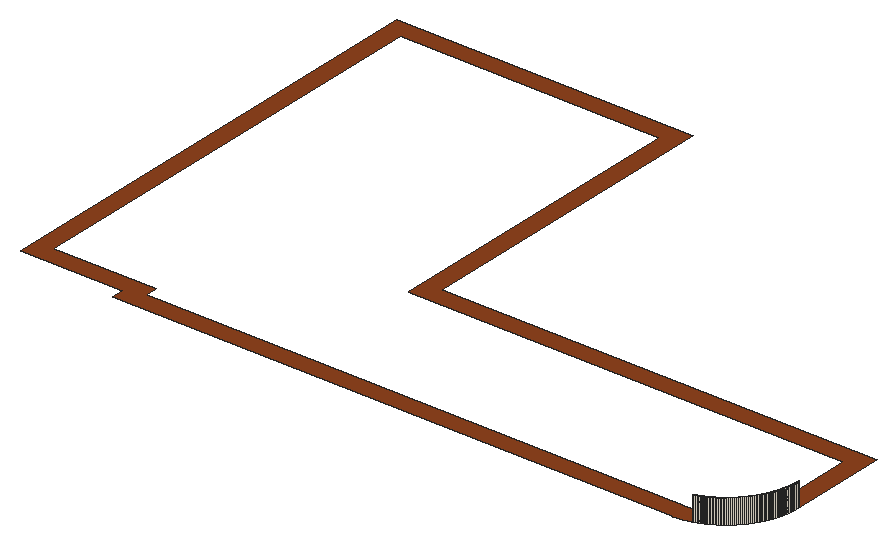
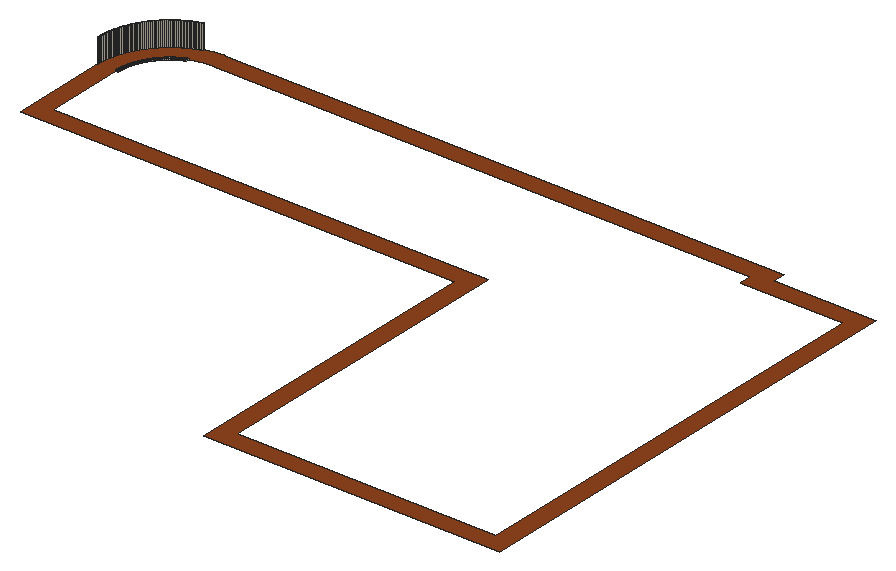
# SketchUp Ruby script. Lengths in inches.
U = 1.inch
M = Sketchup.active_model
def pt(a) = Geom::Point3d.new(a.map { |v| v * U })
def face(e, loops, mat)
  f = e.add_face(loops[0].map { |a| pt(a) })
  loops[1..].each { |l| e.add_face(l.map { |a| pt(a) }).erase! }
  f.material = f.back_material = mat if mat
  f
end
# faces: each face lists its corners as indices into pts; further lists are holes
def faces(e, pts, list, mat = nil) = list.each { |f| face(e, (f[0].is_a?(Array) ? f : [f]).map { |l| l.map { |i| pts[i] } }, mat) }
# xy, xz, yz: faces in a plane at the given z, y or x. An outline is a flat list of corners, or four numbers for a rectangle; further outlines are holes
def ring(l) = l.size == 4 ? [[l[0], l[1]], [l[2], l[1]], [l[2], l[3]], [l[0], l[3]]] : l.each_slice(2).to_a
def flat(e, list, mat, &to3) = list.each { |f| face(e, (f[0].is_a?(Array) ? f : [f]).map { |l| ring(l).map { |u, v| to3.(u, v) } }, mat) }
def xy(e, z, list, mat = nil) = flat(e, list, mat) { |x, y| [x, y, z] }
def xz(e, y, list, mat = nil) = flat(e, list, mat) { |x, z| [x, y, z] }
def yz(e, x, list, mat = nil) = flat(e, list, mat) { |y, z| [x, y, z] }
def lines(e, pts, list) = list.each { |a, b| e.add_line(pt(pts[a]), pt(pts[b])) }
# prism: a flat outline (further loops are holes) pulled along v
def prism(e, loops, v, mat = nil)
  f = face(e, loops, mat); d = Geom::Vector3d.new(v.map { |x| x * U })
  f.pushpull(f.normal.samedirection?(d) ? d.length : -d.length)
end
def box(e, o, s, mat = nil) = prism(e, [[o, [o[0] + s[0], o[1], o[2]], [o[0] + s[0], o[1] + s[1], o[2]], [o[0], o[1] + s[1], o[2]]]], [0, 0, s[2]], mat)
def at(x, y, z, deg = 0) = Geom::Transformation.translation(pt([x, y, z])) * Geom::Transformation.rotation(ORIGIN, Z_AXIS, deg.degrees)
def axes(o, x, y, z) = Geom::Transformation.new([*x, 0, *y, 0, *z, 0, *pt(o).to_a, 1])
def part(name) = M.definitions.add(name)
# library, detail: a bought-in or finely detailed component or shape, given as its bounding box
def library(name, o, s) = part(name).tap { |d| box(d.entities, o, s) }
def detail(e, o, s) = box(e.add_group.entities, o, s)
def put(e, d, t, mat = nil) = e.add_instance(d, t).tap { |i| i.material = mat if mat }
def group(e, t, mat = nil) = e.add_group.tap { |g| g.transformation = t; g.material = mat if mat }.entities
root = M.entities
M.materials.add("0027 AP L140 CRUSHED ICE").color = [241, 233, 217]
M.materials.add("[Wood Fence]").color = [142, 67, 30]
xy(root,120,[[[69,216,69,222,18,222,18,456,165,456,165,300,381,300,381,251.625,380.99,251.25,380.97,250.49,380.95,250.12,380.93,249.74,380.9,249.36,380.875,248.99,380.84,248.61,380.8,248.24,380.76,247.86,380.72,247.49,380.67,247.11,380.61,246.74,380.56,246.37,380.5,246,380.36,245.25,380.29,244.88,380.21,244.52,380.05,243.78,379.96,243.41,379.87,243.05,379.77,242.68,379.57,241.96,379.46,241.59,379.35,241.23,379.24,240.875,379.12,240.52,379,240.16,378.87,239.81,378.74,239.45,378.61,239.1,378.33,238.4,378.1875,238.05,378.04,237.7,377.89,237.36,377.73,237.01,377.25,235.99,377.08,235.66,376.9,235.32,376.73,234.99,376.55,234.66,376.36,234.33,376.18,234,375.99,233.67,375.79,233.35,375.6,233.03,375.4,232.71,375.19,232.39,374.99,232.08,374.77,231.76,374.5625,231.45,374.34,231.15,374.125,230.84,373.9,230.54,373.68,230.23,373.45,229.94,373.21,229.64,372.98,229.34,372.5,228.76,372.25,228.48,372,228.19,371.5,227.63,371.24,227.36,370.98,227.08,370.72,226.8125,370.46,226.54,370.1875,226.28,369.92,226.02,369.64,225.76,369.37,225.5,368.81,225,368.52,224.75,368.24,224.5,367.66,224.02,367.36,223.79,367.06,223.55,366.77,223.32,366.46,223.1,366.16,222.875,365.85,222.66,365.55,222.4375,365.24,222.23,364.92,222.01,364.61,221.81,364.29,221.6,363.97,221.4,363.65,221.21,363.33,221.01,363,220.82,362.67,220.64,362.34,220.45,362.01,220.27,361.68,220.1,361.34,219.92,361.01,219.75,359.99,219.27,359.64,219.11,359.3,218.96,358.95,218.8125,358.6,218.67,357.9,218.39,357.55,218.26,357.19,218.13,356.84,218,356.48,217.88,356.125,217.76,355.77,217.65,355.41,217.54,355.04,217.43,354.32,217.23,353.95,217.13,353.59,217.04,353.22,216.95,352.48,216.79,352.12,216.71,351.75,216.64,351,216.5,350.63,216.44,350.26,216.39,349.89,216.33,349.51,216.28,349.14,216.24,348.76,216.2,348.39,216.16,348.01,216.125,347.64,216.1,347.26,216.07,346.88,216.05,346.51,216.03,345.75,216.01,345.375,216],[78,225,345.28,225,345.57,225.01,345.85,225.01,346.13,225.02,346.41,225.04,346.7,225.05,347.26,225.09,348.38,225.21,349.22,225.33,350.34,225.53,350.61,225.59,351.17,225.71,351.71,225.85,351.99,225.92,352.26,225.99,352.8,226.15,353.07,226.24,353.34,226.32,353.88,226.5,354.15,226.6,354.41,226.69,354.68,226.79,354.9375,226.9,355.2,227,355.98,227.33,356.5,227.57,356.75,227.69,357.01,227.82,357.26,227.94,357.76,228.2,358.01,228.34,358.25,228.48,358.5,228.62,358.74,228.76,358.99,228.91,359.23,229.05,359.47,229.2,359.71,229.36,359.94,229.51,360.18,229.67,360.64,229.99,360.87,230.16,361.1,230.32,361.32,230.49,361.55,230.67,361.77,230.84,362.43,231.38,362.64,231.5625,362.86,231.75,363.07,231.94,363.28,232.125,363.48,232.32,363.6875,232.51,363.89,232.71,364.29,233.11,364.49,233.3125,364.68,233.52,364.875,233.72,365.06,233.93,365.25,234.14,365.4375,234.36,365.62,234.57,366.16,235.23,366.33,235.45,366.51,235.68,366.68,235.9,366.84,236.13,367.01,236.36,367.33,236.82,367.49,237.06,367.64,237.29,367.8,237.53,367.95,237.77,368.09,238.01,368.24,238.26,368.38,238.5,368.52,238.75,368.66,238.99,368.8,239.24,369.06,239.74,369.18,239.99,369.31,240.25,369.43,240.5,369.67,241.02,370,241.8,370.1,242.0625,370.21,242.32,370.31,242.59,370.4,242.85,370.5,243.12,370.68,243.66,370.76,243.93,370.85,244.2,371.01,244.74,371.08,245.01,371.15,245.29,371.29,245.83,371.41,246.39,371.47,246.66,371.67,247.78,371.79,248.62,371.91,249.74,371.95,250.3,371.96,250.59,371.98,250.87,371.99,251.15,371.99,251.43,372,251.72,372,291,156,291,156,447,27,447,27,231,78,231]]],"[Wood Fence]")
yz(root,370.99,[[251.18,120,251.46,120.5]],"0027 AP L140 CRUSHED ICE")
yz(root,371,[[251.73,120,252,120.5]],"0027 AP L140 CRUSHED ICE")
yz(root,371.99,[[251.15,120,251.43,120.5]],"0027 AP L140 CRUSHED ICE")
yz(root,372,[[251.72,120,252,120.5]],"0027 AP L140 CRUSHED ICE")
yz(root,381,[[251.625,120,252,132]],"0027 AP L140 CRUSHED ICE")
p = [[356.125,217.76,132],[355.77,217.65,132],[355.77,217.65,120],[356.125,217.76,120],[356.48,217.88,132],[356.48,217.88,120],
  [356.84,218,132],[356.84,218,120],[357.19,218.13,132],[357.19,218.13,120],[357.55,218.26,132],[357.55,218.26,120],
  [357.9,218.39,132],[357.9,218.39,120],[358.25,218.53,132],[358.25,218.53,120],[358.6,218.67,132],[358.6,218.67,120],
  [358.95,218.8125,132],[358.95,218.8125,120],[359.3,218.96,132],[359.3,218.96,120],[359.64,219.11,132],[359.64,219.11,120],
  [359.99,219.27,132],[359.99,219.27,120],[360.33,219.43,132],[360.33,219.43,120],[360.67,219.59,132],[360.67,219.59,120],
  [361.01,219.75,132],[361.01,219.75,120],[361.34,219.92,132],[361.34,219.92,120],[361.68,220.1,132],[361.68,220.1,120],
  [362.01,220.27,132],[362.01,220.27,120],[362.34,220.45,132],[362.34,220.45,120],[362.67,220.64,132],[362.67,220.64,120],
  [363,220.82,132],[363,220.82,120],[363.33,221.01,132],[363.33,221.01,120],[363.65,221.21,132],[363.65,221.21,120],
  [363.97,221.4,132],[363.97,221.4,120],[364.29,221.6,132],[364.29,221.6,120],[364.61,221.81,132],[364.61,221.81,120],
  [364.92,222.01,132],[364.92,222.01,120],[365.24,222.23,132],[365.24,222.23,120],[365.55,222.4375,132],[365.55,222.4375,120],
  [365.85,222.66,132],[365.85,222.66,120],[366.16,222.875,132],[366.16,222.875,120],[366.46,223.1,132],[366.46,223.1,120],
  [366.77,223.32,132],[366.77,223.32,120],[367.06,223.55,132],[367.06,223.55,120],[367.36,223.79,132],[367.36,223.79,120],
  [367.66,224.02,132],[367.66,224.02,120],[367.95,224.26,132],[367.95,224.26,120],[368.24,224.5,132],[368.24,224.5,120],
  [368.52,224.75,132],[368.52,224.75,120],[368.81,225,132],[368.81,225,120],[369.09,225.25,132],[369.09,225.25,120],
  [369.37,225.5,132],[369.37,225.5,120],[369.64,225.76,132],[369.64,225.76,120],[369.92,226.02,132],[369.92,226.02,120],
  [370.1875,226.28,132],[370.1875,226.28,120],[370.46,226.54,132],[370.46,226.54,120],[370.72,226.8125,132],[370.72,226.8125,120],
  [370.98,227.08,132],[370.98,227.08,120],[371.24,227.36,132],[371.24,227.36,120],[355.98,227.33,120],[355.72,227.22,120],
  [355.72,227.22,120.5],[355.98,227.33,120.5],[356.24,227.45,120],[356.24,227.45,120.5],[371.5,227.63,132],[371.5,227.63,120],
  [356.5,227.57,120],[356.5,227.57,120.5],[356.75,227.69,120],[356.75,227.69,120.5],[371.75,227.91,132],[371.75,227.91,120],
  [357.01,227.82,120],[357.01,227.82,120.5],[357.26,227.94,120],[357.26,227.94,120.5],[357.51,228.07,120],[357.51,228.07,120.5],
  [372,228.19,132],[372,228.19,120],[357.76,228.2,120],[357.76,228.2,120.5],[355.58,228.25,120],[355.82,228.36,120],
  [355.82,228.36,120.5],[355.58,228.25,120.5],[358.01,228.34,120],[358.01,228.34,120.5],[372.25,228.48,132],[372.25,228.48,120],
  [358.25,228.48,120],[358.25,228.48,120.5],[356.07,228.47,120],[356.07,228.47,120.5],[356.32,228.59,120],[356.32,228.59,120.5],
  [358.5,228.62,120],[358.5,228.62,120.5],[372.5,228.76,132],[372.5,228.76,120],[356.5625,228.71,120],[356.5625,228.71,120.5],
  [358.74,228.76,120],[358.74,228.76,120.5],[356.8,228.83,120],[356.8,228.83,120.5],[357.05,228.96,120],[357.05,228.96,120.5],
  [358.99,228.91,120],[358.99,228.91,120.5],[372.74,229.05,132],[372.74,229.05,120],[359.23,229.05,120],[359.23,229.05,120.5],
  [357.29,229.09,120],[357.29,229.09,120.5],[357.53,229.22,120],[357.53,229.22,120.5],[359.47,229.2,120],[359.47,229.2,120.5],
  [372.98,229.34,132],[372.98,229.34,120],[357.76,229.35,120],[357.76,229.35,120.5],[359.71,229.36,120],[359.71,229.36,120.5],
  [358,229.48,120],[358,229.48,120.5],[373.21,229.64,132],[373.21,229.64,120],[359.94,229.51,120],[359.94,229.51,120.5],
  [358.24,229.62,120],[358.24,229.62,120.5],[360.18,229.67,120],[360.18,229.67,120.5],[358.47,229.76,120],[358.47,229.76,120.5],
  [373.45,229.94,132],[373.45,229.94,120],[360.41,229.83,120],[360.41,229.83,120.5],[358.7,229.9,120],[358.7,229.9,120.5],
  [360.64,229.99,120],[360.64,229.99,120.5],[358.93,230.05,120],[358.93,230.05,120.5],[373.68,230.23,132],[373.68,230.23,120],
  [359.16,230.19,120],[359.16,230.19,120.5],[360.87,230.16,120],[360.87,230.16,120.5],[359.39,230.34,120],[359.39,230.34,120.5],
  [361.1,230.32,120],[361.1,230.32,120.5],[373.9,230.54,132],[373.9,230.54,120],[359.61,230.5,120],[359.61,230.5,120.5],
  [361.32,230.49,120],[361.32,230.49,120.5],[359.84,230.65,120],[359.84,230.65,120.5],[361.55,230.67,120],[361.55,230.67,120.5],
  [374.125,230.84,132],[374.125,230.84,120],[360.0625,230.81,120],[360.0625,230.81,120.5],[361.77,230.84,120],[361.77,230.84,120.5],
  [360.28,230.97,120],[360.28,230.97,120.5],[361.99,231.02,120],[361.99,231.02,120.5],[374.34,231.15,132],[374.34,231.15,120],
  [360.5,231.125,120],[360.5,231.125,120.5],[362.21,231.2,120],[362.21,231.2,120.5],[360.72,231.29,120],[360.72,231.29,120.5],
  [374.5625,231.45,132],[374.5625,231.45,120],[362.43,231.38,120],[362.43,231.38,120.5],[360.9375,231.46,120],[360.9375,231.46,120.5],
  [362.64,231.5625,120],[362.64,231.5625,120.5],[361.15,231.625,120],[361.15,231.625,120.5],[374.77,231.76,132],[374.77,231.76,120],
  [361.36,231.79,120],[361.36,231.79,120.5],[362.86,231.75,120],[362.86,231.75,120.5],[363.07,231.94,120],[363.07,231.94,120.5],
  [361.57,231.97,120],[361.57,231.97,120.5],[374.99,232.08,132],[374.99,232.08,120],[363.28,232.125,120],[363.28,232.125,120.5],
  [361.78,232.14,120],[361.78,232.14,120.5],[361.99,232.32,120],[361.99,232.32,120.5],[363.48,232.32,120],[363.48,232.32,120.5],
  [375.19,232.39,132],[375.19,232.39,120],[362.19,232.5,120],[362.19,232.5,120.5],[363.6875,232.51,120],[363.6875,232.51,120.5],
  [375.4,232.71,132],[375.4,232.71,120],[362.4,232.68,120],[362.4,232.68,120.5],[363.89,232.71,120],[363.89,232.71,120.5],
  [362.6,232.86,120],[362.6,232.86,120.5],[364.09,232.91,120],[364.09,232.91,120.5],[375.6,233.03,132],[375.6,233.03,120],
  [362.8,233.05,120],[362.8,233.05,120.5],[364.29,233.11,120],[364.29,233.11,120.5],[363,233.23,120],[363,233.23,120.5],
  [375.79,233.35,132],[375.79,233.35,120],[364.49,233.3125,120],[364.49,233.3125,120.5],[363.19,233.42,120],[363.19,233.42,120.5],
  [364.68,233.52,120],[364.68,233.52,120.5],[363.38,233.62,120],[363.38,233.62,120.5],[375.99,233.67,132],[375.99,233.67,120],
  [364.875,233.72,120],[364.875,233.72,120.5],[363.58,233.81,120],[363.58,233.81,120.5],[365.06,233.93,120],[365.06,233.93,120.5],
  [376.18,234,132],[376.18,234,120],[363.77,234,120],[363.77,234,120.5],[365.25,234.14,120],[365.25,234.14,120.5],
  [363.95,234.2,120],[363.95,234.2,120.5],[376.36,234.33,132],[376.36,234.33,120],[365.4375,234.36,120],[365.4375,234.36,120.5],
  [364.14,234.4,120],[364.14,234.4,120.5],[376.55,234.66,132],[376.55,234.66,120],[364.32,234.6,120],[364.32,234.6,120.5],
  [365.62,234.57,120],[365.62,234.57,120.5],[364.5,234.81,120],[364.5,234.81,120.5],[365.8,234.79,120],[365.8,234.79,120.5],
  [376.73,234.99,132],[376.73,234.99,120],[364.68,235.01,120],[364.68,235.01,120.5],[365.98,235.01,120],[365.98,235.01,120.5],
  [364.86,235.22,120],[364.86,235.22,120.5],[366.16,235.23,120],[366.16,235.23,120.5],[376.9,235.32,132],[376.9,235.32,120],
  [365.03,235.43,120],[365.03,235.43,120.5],[366.33,235.45,120],[366.33,235.45,120.5],[377.08,235.66,132],[377.08,235.66,120],
  [365.21,235.64,120],[365.21,235.64,120.5],[366.51,235.68,120],[366.51,235.68,120.5],[365.375,235.85,120],[365.375,235.85,120.5],
  [366.68,235.9,120],[366.68,235.9,120.5],[377.25,235.99,132],[377.25,235.99,120],[365.54,236.0625,120],[365.54,236.0625,120.5],
  [366.84,236.13,120],[366.84,236.13,120.5],[377.41,236.33,132],[377.41,236.33,120],[365.71,236.28,120],[365.71,236.28,120.5],
  [367.01,236.36,120],[367.01,236.36,120.5],[365.875,236.5,120],[365.875,236.5,120.5],[377.57,236.67,132],[377.57,236.67,120],
  [367.17,236.59,120],[367.17,236.59,120.5],[366.03,236.72,120],[366.03,236.72,120.5],[367.33,236.82,120],[367.33,236.82,120.5],
  [366.19,236.9375,120],[366.19,236.9375,120.5],[377.73,237.01,132],[377.73,237.01,120],[367.49,237.06,120],[367.49,237.06,120.5],
  [366.35,237.16,120],[366.35,237.16,120.5],[377.89,237.36,132],[377.89,237.36,120],[367.64,237.29,120],[367.64,237.29,120.5],
  [366.5,237.39,120],[366.5,237.39,120.5],[367.8,237.53,120],[367.8,237.53,120.5],[366.66,237.61,120],[366.66,237.61,120.5],
  [378.04,237.7,132],[378.04,237.7,120],[367.95,237.77,120],[367.95,237.77,120.5],[366.81,237.84,120],[366.81,237.84,120.5],
  [378.1875,238.05,132],[378.1875,238.05,120],[366.95,238.07,120],[366.95,238.07,120.5],[368.09,238.01,120],[368.09,238.01,120.5],
  [368.24,238.26,120],[368.24,238.26,120.5],[378.33,238.4,132],[378.33,238.4,120],[367.1,238.3,120],[367.1,238.3,120.5],
  [367.24,238.53,120],[367.24,238.53,120.5],[368.38,238.5,120],[368.38,238.5,120.5],[378.47,238.75,132],[378.47,238.75,120],
  [367.38,238.76,120],[367.38,238.76,120.5],[368.52,238.75,120],[368.52,238.75,120.5],[368.66,238.99,120],[368.66,238.99,120.5],
  [378.61,239.1,132],[378.61,239.1,120],[367.52,239,120],[367.52,239,120.5],[367.65,239.24,120],[367.65,239.24,120.5],
  [368.8,239.24,120],[368.8,239.24,120.5],[378.74,239.45,132],[378.74,239.45,120],[367.78,239.47,120],[367.78,239.47,120.5],
  [368.93,239.49,120],[368.93,239.49,120.5],[367.91,239.71,120],[367.91,239.71,120.5],[369.06,239.74,120],[369.06,239.74,120.5],
  [378.87,239.81,132],[378.87,239.81,120],[368.04,239.95,120],[368.04,239.95,120.5],[369.18,239.99,120],[369.18,239.99,120.5],
  [379,240.16,132],[379,240.16,120],[368.17,240.2,120],[368.17,240.2,120.5],[369.31,240.25,120],[369.31,240.25,120.5],
  [368.29,240.4375,120],[368.29,240.4375,120.5],[369.43,240.5,120],[369.43,240.5,120.5],[379.12,240.52,132],[379.12,240.52,120],
  [368.41,240.68,120],[368.41,240.68,120.5],[369.55,240.76,120],[369.55,240.76,120.5],[379.24,240.875,132],[379.24,240.875,120],
  [368.53,240.93,120],[368.53,240.93,120.5],[369.67,241.02,120],[369.67,241.02,120.5],[368.64,241.18,120],[368.64,241.18,120.5],
  [379.35,241.23,132],[379.35,241.23,120],[369.78,241.28,120],[369.78,241.28,120.5],[368.75,241.42,120],[368.75,241.42,120.5],
  [379.46,241.59,132],[379.46,241.59,120],[369.89,241.54,120],[369.89,241.54,120.5],[368.86,241.67,120],[368.86,241.67,120.5],
  [370,241.8,120],[370,241.8,120.5],[379.57,241.96,132],[379.57,241.96,120],[368.97,241.92,120],[368.97,241.92,120.5],
  [370.1,242.0625,120],[370.1,242.0625,120.5],[369.07,242.18,120],[369.07,242.18,120.5],[379.67,242.32,132],[379.67,242.32,120],
  [370.21,242.32,120],[370.21,242.32,120.5],[369.17,242.43,120],[369.17,242.43,120.5],[370.31,242.59,120],[370.31,242.59,120.5],
  [379.77,242.68,132],[379.77,242.68,120],[369.27,242.68,120],[369.27,242.68,120.5],[370.4,242.85,120],[370.4,242.85,120.5],
  [369.37,242.9375,120],[369.37,242.9375,120.5],[379.87,243.05,132],[379.87,243.05,120],[369.46,243.19,120],[369.46,243.19,120.5],
  [370.5,243.12,120],[370.5,243.12,120.5],[379.96,243.41,132],[379.96,243.41,120],[370.59,243.39,120],[370.59,243.39,120.5],
  [369.55,243.45,120],[369.55,243.45,120.5],[369.64,243.71,120],[369.64,243.71,120.5],[370.68,243.66,120],[370.68,243.66,120.5],
  [380.05,243.78,132],[380.05,243.78,120],[369.73,243.97,120],[369.73,243.97,120.5],[370.76,243.93,120],[370.76,243.93,120.5],
  [380.13,244.15,132],[380.13,244.15,120],[370.85,244.2,120],[370.85,244.2,120.5],[369.81,244.22,120],[369.81,244.22,120.5],
  [380.21,244.52,132],[380.21,244.52,120],[369.89,244.49,120],[369.89,244.49,120.5],[370.93,244.47,120],[370.93,244.47,120.5],
  [369.97,244.75,120],[369.97,244.75,120.5],[371.01,244.74,120],[371.01,244.74,120.5],[380.29,244.88,132],[380.29,244.88,120],
  [370.04,245.01,120],[370.04,245.01,120.5],[371.08,245.01,120],[371.08,245.01,120.5],[380.36,245.25,132],[380.36,245.25,120],
  [370.11,245.27,120],[370.11,245.27,120.5],[371.15,245.29,120],[371.15,245.29,120.5],[370.18,245.53,120],[370.18,245.53,120.5],
  [371.22,245.56,120],[371.22,245.56,120.5],[380.43,245.625,132],[380.43,245.625,120],[370.25,245.8,120],[370.25,245.8,120.5],
  [371.29,245.83,120],[371.29,245.83,120.5],[380.5,246,132],[380.5,246,120],[370.3125,246.0625,120],[370.3125,246.0625,120.5],
  [371.35,246.11,120],[371.35,246.11,120.5],[380.56,246.37,132],[380.56,246.37,120],[370.375,246.33,120],[370.375,246.33,120.5],
  [371.41,246.39,120],[371.41,246.39,120.5],[370.43,246.59,120],[370.43,246.59,120.5],[371.47,246.66,120],[371.47,246.66,120.5],
  [380.61,246.74,132],[380.61,246.74,120],[370.49,246.86,120],[370.49,246.86,120.5],[371.52,246.94,120],[371.52,246.94,120.5],
  [380.67,247.11,132],[380.67,247.11,120],[370.54,247.13,120],[370.54,247.13,120.5],[371.57,247.22,120],[371.57,247.22,120.5],
  [370.59,247.4,120],[370.59,247.4,120.5],[380.72,247.49,132],[380.72,247.49,120],[371.62,247.5,120],[371.62,247.5,120.5],
  [370.64,247.66,120],[370.64,247.66,120.5],[371.67,247.78,120],[371.67,247.78,120.5],[380.76,247.86,132],[380.76,247.86,120],
  [370.68,247.93,120],[370.68,247.93,120.5],[371.71,248.06,120],[371.71,248.06,120.5],[370.72,248.2,120],[370.72,248.2,120.5],
  [380.8,248.24,132],[380.8,248.24,120],[371.75,248.34,120],[371.75,248.34,120.5],[370.76,248.47,120],[370.76,248.47,120.5],
  [380.84,248.61,132],[380.84,248.61,120],[371.79,248.62,120],[371.79,248.62,120.5],[370.79,248.74,120],[370.79,248.74,120.5],
  [371.82,248.9,120],[371.82,248.9,120.5],[380.875,248.99,132],[380.875,248.99,120],[370.83,249.01,120],[370.83,249.01,120.5],
  [371.85,249.18,120],[371.85,249.18,120.5],[370.86,249.28,120],[370.86,249.28,120.5],[380.9,249.36,132],[380.9,249.36,120],
  [371.88,249.46,120],[371.88,249.46,120.5],[370.88,249.55,120],[370.88,249.55,120.5],[380.93,249.74,132],[380.93,249.74,120],
  [371.91,249.74,120],[371.91,249.74,120.5],[370.91,249.82,120],[370.91,249.82,120.5],[371.93,250.02,120],[371.93,250.02,120.5],
  [380.95,250.12,132],[380.95,250.12,120],[370.93,250.1,120],[370.93,250.1,120.5],[371.95,250.3,120],[371.95,250.3,120.5],
  [370.95,250.37,120],[370.95,250.37,120.5],[380.97,250.49,132],[380.97,250.49,120],[371.96,250.59,120],[371.96,250.59,120.5],
  [370.96,250.64,120],[370.96,250.64,120.5],[380.98,250.87,132],[380.98,250.87,120],[370.98,250.91,120],[370.98,250.91,120.5],
  [371.98,250.87,120],[371.98,250.87,120.5],[370.99,251.18,120],[370.99,251.18,120.5],[371.99,251.15,120],[371.99,251.15,120.5],
  [380.99,251.25,132],[380.99,251.25,120],[381,251.625,132],[381,251.625,120],[372,251.72,120],[371.99,251.43,120],
  [371.99,251.43,120.5],[372,251.72,120.5],[370.99,251.46,120],[371,251.73,120],[371,251.73,120.5],[370.99,251.46,120.5]]
faces(root,p,[[0,1,2,3],[4,0,3,5],[6,4,5,7],[8,6,7,9],[10,8,9,11],[12,10,11,13],[14,12,13,15],[16,14,15,17],
  [18,16,17,19],[20,18,19,21],[22,20,21,23],[24,22,23,25],[26,24,25,27],[28,26,27,29],[30,28,29,31],[32,30,31,33],
  [34,32,33,35],[36,34,35,37],[38,36,37,39],[40,38,39,41],[42,40,41,43],[44,42,43,45],[46,44,45,47],[48,46,47,49],
  [50,48,49,51],[52,50,51,53],[54,52,53,55],[56,54,55,57],[58,56,57,59],[60,58,59,61],[62,60,61,63],[64,62,63,65],
  [66,64,65,67],[68,66,67,69],[70,68,69,71],[72,70,71,73],[74,72,73,75],[76,74,75,77],[78,76,77,79],[80,78,79,81],
  [82,80,81,83],[84,82,83,85],[86,84,85,87],[88,86,87,89],[90,88,89,91],[92,90,91,93],[94,92,93,95],[96,94,95,97],
  [98,96,97,99],[100,101,102,103],[104,100,103,105],[106,98,99,107],[108,104,105,109],[110,108,109,111],[112,106,107,113],[114,110,111,115],
  [116,114,115,117],[118,116,117,119],[120,112,113,121],[122,118,119,123],[124,125,126,127],[128,122,123,129],[130,120,121,131],[132,128,129,133],
  [125,134,135,126],[134,136,137,135],[138,132,133,139],[140,130,131,141],[136,142,143,137],[144,138,139,145],[142,146,147,143],[146,148,149,147],
  [150,144,145,151],[152,140,141,153],[154,150,151,155],[148,156,157,149],[156,158,159,157],[160,154,155,161],[162,152,153,163],[158,164,165,159],
  [166,160,161,167],[164,168,169,165],[170,162,163,171],[172,166,167,173],[168,174,175,169],[176,172,173,177],[174,178,179,175],[180,170,171,181],
  [182,176,177,183],[178,184,185,179],[186,182,183,187],[184,188,189,185],[190,180,181,191],[188,192,193,189],[194,186,187,195],[192,196,197,193],
  [198,194,195,199],[200,190,191,201],[196,202,203,197],[204,198,199,205],[202,206,207,203],[208,204,205,209],[210,200,201,211],[206,212,213,207],
  [214,208,209,215],[212,216,217,213],[218,214,215,219],[220,210,211,221],[216,222,223,217],[224,218,219,225],[222,226,227,223],[228,220,221,229],
  [230,224,225,231],[226,232,233,227],[234,230,231,235],[232,236,237,233],[238,228,229,239],[236,240,241,237],[242,234,235,243],[244,242,243,245],
  [240,246,247,241],[248,238,239,249],[250,244,245,251],[246,252,253,247],[252,254,255,253],[256,250,251,257],[258,248,249,259],[254,260,261,255],
  [262,256,257,263],[264,258,259,265],[260,266,267,261],[268,262,263,269],[266,270,271,267],[272,268,269,273],[274,264,265,275],[270,276,277,271],
  [278,272,273,279],[276,280,281,277],[282,274,275,283],[284,278,279,285],[280,286,287,281],[288,284,285,289],[286,290,291,287],[292,282,283,293],
  [294,288,289,295],[290,296,297,291],[298,294,295,299],[300,292,293,301],[296,302,303,297],[304,298,299,305],[302,306,307,303],[308,300,301,309],
  [310,304,305,311],[306,312,313,307],[314,308,309,315],[312,316,317,313],[318,310,311,319],[316,320,321,317],[322,318,319,323],[324,314,315,325],
  [320,326,327,321],[328,322,323,329],[326,330,331,327],[332,328,329,333],[334,324,325,335],[330,336,337,331],[338,332,333,339],[340,334,335,341],
  [336,342,343,337],[344,338,339,345],[342,346,347,343],[348,344,345,349],[350,340,341,351],[346,352,353,347],[354,348,349,355],[356,350,351,357],
  [352,358,359,353],[360,354,355,361],[358,362,363,359],[364,356,357,365],[366,360,361,367],[362,368,369,363],[370,366,367,371],[368,372,373,369],
  [374,364,365,375],[376,370,371,377],[372,378,379,373],[380,374,375,381],[382,376,377,383],[378,384,385,379],[386,382,383,387],[384,388,389,385],
  [390,380,381,391],[392,386,387,393],[388,394,395,389],[396,390,391,397],[394,398,399,395],[400,392,393,401],[402,400,401,403],[404,396,397,405],
  [398,406,407,399],[406,408,409,407],[410,402,403,411],[412,404,405,413],[408,414,415,409],[416,410,411,417],[418,416,417,419],[420,412,413,421],
  [414,422,423,415],[422,424,425,423],[426,418,419,427],[428,420,421,429],[424,430,431,425],[432,426,427,433],[430,434,435,431],[436,432,433,437],
  [438,428,429,439],[434,440,441,435],[442,436,437,443],[444,438,439,445],[440,446,447,441],[448,442,443,449],[446,450,451,447],[452,448,449,453],
  [454,444,445,455],[450,456,457,451],[458,452,453,459],[460,454,455,461],[456,462,463,457],[464,458,459,465],[462,466,467,463],[468,460,461,469],
  [470,464,465,471],[466,472,473,467],[474,468,469,475],[476,470,471,477],[472,478,479,473],[480,476,477,481],[482,474,475,483],[478,484,485,479],
  [486,480,481,487],[484,488,489,485],[490,482,483,491],[492,486,487,493],[488,494,495,489],[496,492,493,497],[498,490,491,499],[494,500,501,495],
  [502,496,497,503],[500,504,505,501],[506,498,499,507],[504,508,509,505],[510,502,503,511],[512,506,507,513],[514,510,511,515],[508,516,517,509],
  [516,518,519,517],[520,514,515,521],[522,512,513,523],[518,524,525,519],[526,520,521,527],[528,522,523,529],[530,526,527,531],[524,532,533,525],
  [534,528,529,535],[532,536,537,533],[538,530,531,539],[536,540,541,537],[542,538,539,543],[544,534,535,545],[540,546,547,541],[548,542,543,549],
  [550,544,545,551],[546,552,553,547],[554,548,549,555],[552,556,557,553],[558,554,555,559],[560,550,551,561],[556,562,563,557],[564,558,559,565],
  [566,560,561,567],[562,568,569,563],[570,564,565,571],[572,566,567,573],[568,574,575,569],[576,570,571,577],[574,578,579,575],[580,576,577,581],
  [582,572,573,583],[578,584,585,579],[586,580,581,587],[588,582,583,589],[584,590,591,585],[592,586,587,593],[590,594,595,591],[596,588,589,597],
  [598,592,593,599],[594,600,601,595],[602,598,599,603],[604,596,597,605],[600,606,607,601],[608,602,603,609],[606,610,611,607],[612,604,605,613],
  [614,608,609,615],[610,616,617,611],[618,612,613,619],[620,614,615,621],[616,622,623,617],[624,620,621,625],[626,618,619,627],[622,628,629,623],
  [630,624,625,631],[628,632,633,629],[634,626,627,635],[636,630,631,637],[632,638,639,633],[640,634,635,641],[642,636,637,643],[638,644,645,639],
  [646,642,643,647],[648,640,641,649],[644,650,651,645],[652,646,647,653],[650,654,655,651],[656,648,649,657],[658,652,653,659],[654,660,661,655],
  [662,656,657,663],[660,664,665,661],[666,658,659,667],[664,668,669,665],[670,666,667,671],[672,662,663,673],[674,672,673,675],[676,677,678,679],
  [680,681,682,683]],"0027 AP L140 CRUSHED ICE")
